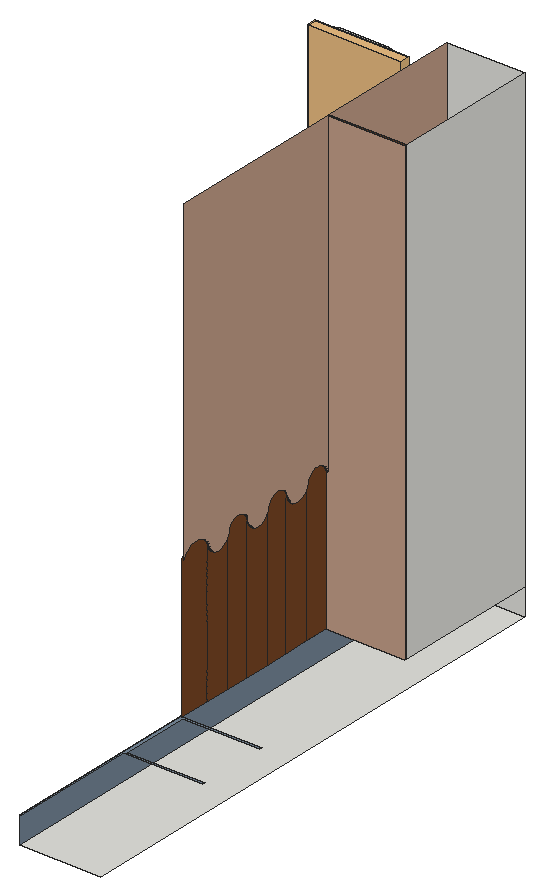
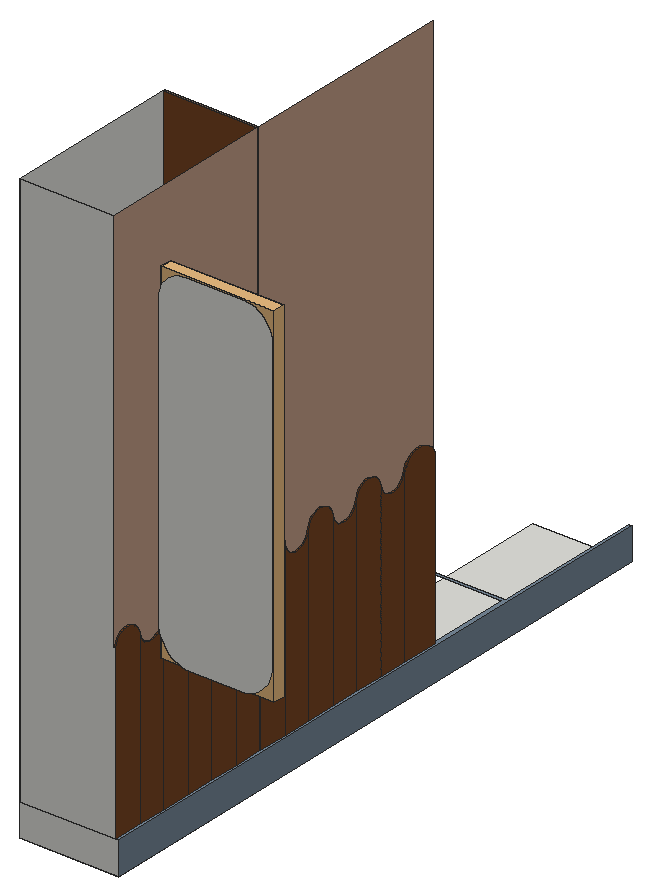
# SketchUp Ruby script. Lengths in inches.
U = 1.inch
M = Sketchup.active_model
def pt(a) = Geom::Point3d.new(a.map { |v| v * U })
def face(e, loops, mat)
  f = e.add_face(loops[0].map { |a| pt(a) })
  loops[1..].each { |l| e.add_face(l.map { |a| pt(a) }).erase! }
  f.material = f.back_material = mat if mat
  f
end
# faces: each face lists its corners as indices into pts; further lists are holes
def faces(e, pts, list, mat = nil) = list.each { |f| face(e, (f[0].is_a?(Array) ? f : [f]).map { |l| l.map { |i| pts[i] } }, mat) }
# xy, xz, yz: faces in a plane at the given z, y or x. An outline is a flat list of corners, or four numbers for a rectangle; further outlines are holes
def ring(l) = l.size == 4 ? [[l[0], l[1]], [l[2], l[1]], [l[2], l[3]], [l[0], l[3]]] : l.each_slice(2).to_a
def flat(e, list, mat, &to3) = list.each { |f| face(e, (f[0].is_a?(Array) ? f : [f]).map { |l| ring(l).map { |u, v| to3.(u, v) } }, mat) }
def xy(e, z, list, mat = nil) = flat(e, list, mat) { |x, y| [x, y, z] }
def xz(e, y, list, mat = nil) = flat(e, list, mat) { |x, z| [x, y, z] }
def yz(e, x, list, mat = nil) = flat(e, list, mat) { |y, z| [x, y, z] }
def lines(e, pts, list) = list.each { |a, b| e.add_line(pt(pts[a]), pt(pts[b])) }
# prism: a flat outline (further loops are holes) pulled along v
def prism(e, loops, v, mat = nil)
  f = face(e, loops, mat); d = Geom::Vector3d.new(v.map { |x| x * U })
  f.pushpull(f.normal.samedirection?(d) ? d.length : -d.length)
end
def box(e, o, s, mat = nil) = prism(e, [[o, [o[0] + s[0], o[1], o[2]], [o[0] + s[0], o[1] + s[1], o[2]], [o[0], o[1] + s[1], o[2]]]], [0, 0, s[2]], mat)
def at(x, y, z, deg = 0) = Geom::Transformation.translation(pt([x, y, z])) * Geom::Transformation.rotation(ORIGIN, Z_AXIS, deg.degrees)
def axes(o, x, y, z) = Geom::Transformation.new([*x, 0, *y, 0, *z, 0, *pt(o).to_a, 1])
def part(name) = M.definitions.add(name)
# library, detail: a bought-in or finely detailed component or shape, given as its bounding box
def library(name, o, s) = part(name).tap { |d| box(d.entities, o, s) }
def detail(e, o, s) = box(e.add_group.entities, o, s)
def put(e, d, t, mat = nil) = e.add_instance(d, t).tap { |i| i.material = mat if mat }
def group(e, t, mat = nil) = e.add_group.tap { |g| g.transformation = t; g.material = mat if mat }.entities
root = M.entities
M.materials.add("[0009_Linen]").color = [197, 160, 138]
M.materials.add("[0110_LightSlateGray]1").color = [119, 136, 153]
M.materials.add("[Wood Veneer 01]").color = [120, 70, 37]
xy(root,6.125,[[535.07,78.14,558.07,228.1]])
xy(root,13.75,[[535.07,78.14,535.64,78.14,535.64,114.14,558.07,114.14,558.07,114.74,536.14,114.74,536.14,134.3125,558.07,134.3125,558.07,134.91,535.64,134.91,535.64,185.66,558.07,185.66,558.07,186.26,535.64,186.26,535.64,228.1,535.07,228.1]],"[0110_LightSlateGray]1")
xz(root,185.66,[[535.64,13.75,535.64,53.75,536.14,53.75,536.14,144.125,558.07,144.125,558.07,13.75]],"[0009_Linen]")
xz(root,186.26,[[535.64,13.75,558.07,13.75,558.07,144.125,536.14,144.125,536.14,53.75,535.64,53.75]],"[Wood Veneer 01]")
xz(root,228.1,[[535.07,6.125,558.07,13.75],[535.64,13.75,535.64,53.75,536.14,53.75,536.14,144.125,558.07,144.125,558.07,13.75],[505.51,54.9375,504.65,55.14,503.8125,55.44,503.02,55.84,502.28,56.32,501.6,56.89,500.99,57.54,500.46,58.25,500.01,59.01,499.66,59.83,499.4,60.68,499.25,61.55,499.2,62.4375,499.2,130.5625,499.25,131.4,499.42,132.23,499.6875,133.03,500.06,133.78,500.53,134.48,501.08,135.11,501.72,135.67,502.42,136.14,503.17,136.51,503.97,136.78,504.79,136.94,505.64,137,519.39,137,520.21,136.94,521.03,136.78,521.8125,136.5,522.55,136.13,523.24,135.66,523.85,135.1,524.38,134.46,524.83,133.76,525.17,133.01,525.42,132.21,525.55,131.39,525.57,130.5625,525.57,62.4375,525.52,61.5625,525.37,60.7,525.12,59.85,524.78,59.05,524.34,58.28,523.83,57.58,523.23,56.93,522.5625,56.36,521.84,55.87,521.06,55.47,520.24,55.15,519.39,54.9375]])
yz(root,535.07,[[78.14,6.125,228.1,13.75]],"[0110_LightSlateGray]1")
yz(root,535.64,[[134.91,13.75,134.91,53.75,135.34,54.59,135.92,55.32,136.63,55.93,137.46,56.38,138.35,56.66,139.29,56.75,140.22,56.66,141.12,56.38,141.9375,55.93,142.66,55.32,143.24,54.59,143.66,53.75,143.66,13.75],[143.66,13.75,143.66,53.75,143.89,52.95,144.29,52.22,144.86,51.6,145.55,51.14,146.33,50.85,147.16,50.75,147.99,50.85,148.77,51.14,149.47,51.6,150.03,52.22,150.4375,52.95,150.66,53.75,150.66,13.75],[150.66,13.75,150.66,53.75,150.89,54.55,151.29,55.28,151.86,55.9,152.55,56.36,153.33,56.65,154.16,56.75,154.99,56.65,155.77,56.36,156.47,55.9,157.03,55.28,157.4375,54.55,157.66,53.75,157.66,13.75],[157.66,13.75,157.66,53.75,157.89,52.95,158.29,52.22,158.86,51.6,159.55,51.14,160.33,50.85,161.16,50.75,161.99,50.85,162.77,51.14,163.47,51.6,164.03,52.22,164.4375,52.95,164.66,53.75,164.66,13.75],[164.66,13.75,164.66,53.75,164.89,54.55,165.29,55.28,165.86,55.9,166.55,56.36,167.33,56.65,168.16,56.75,168.99,56.65,169.77,56.36,170.47,55.9,171.03,55.28,171.4375,54.55,171.66,53.75,171.66,13.75],
  [171.66,13.75,171.66,53.75,171.89,52.95,172.29,52.22,172.86,51.6,173.55,51.14,174.33,50.85,175.16,50.75,175.99,50.85,176.77,51.14,177.47,51.6,178.03,52.22,178.4375,52.95,178.66,53.75,178.66,13.75],[178.66,13.75,178.66,53.75,178.89,54.55,179.29,55.28,179.86,55.9,180.55,56.36,181.33,56.65,182.16,56.75,182.99,56.65,183.77,56.36,184.47,55.9,185.03,55.28,185.4375,54.55,185.66,53.75,185.66,13.75],[186.26,13.75,186.26,53.75,186.47,52.95,186.86,52.22,187.41,51.61,188.09,51.14,188.86,50.85,189.68,50.75,190.5,50.85,191.28,51.14,191.96,51.61,192.51,52.22,192.9,52.95,193.1,53.75,193.1,13.75],[193.1,13.75,193.1,53.75,193.33,54.55,193.73,55.28,194.3,55.9,194.99,56.36,195.77,56.65,196.6,56.75,197.43,56.65,198.22,56.36,198.91,55.9,199.47,55.28,199.88,54.55,200.1,53.75,200.1,13.75],[200.1,13.75,200.1,53.75,200.33,52.95,200.73,52.22,201.3,51.6,201.99,51.14,202.77,50.85,203.6,50.75,204.43,50.85,205.22,51.14,205.91,51.6,206.47,52.22,206.88,52.95,207.1,53.75,207.1,13.75],
  [207.1,13.75,207.1,53.75,207.33,54.55,207.73,55.28,208.3,55.9,208.99,56.36,209.77,56.65,210.6,56.75,211.43,56.65,212.22,56.36,212.91,55.9,213.47,55.28,213.88,54.55,214.1,53.75,214.1,13.75],[214.1,13.75,214.1,53.75,214.33,52.95,214.73,52.22,215.3,51.6,215.99,51.14,216.77,50.85,217.6,50.75,218.43,50.85,219.22,51.14,219.91,51.6,220.47,52.22,220.88,52.95,221.1,53.75,221.1,13.75],[221.1,13.75,221.1,53.75,221.33,54.55,221.73,55.28,222.3,55.9,222.99,56.36,223.77,56.65,224.6,56.75,225.43,56.65,226.22,56.36,226.91,55.9,227.47,55.28,227.88,54.55,228.1,53.75,228.1,13.75]],"[Wood Veneer 01]")
yz(root,536.14,[[147.16,50.75,146.33,50.85,145.55,51.14,144.86,51.6,144.29,52.22,143.89,52.95,143.66,53.75,143.24,54.59,142.66,55.32,141.9375,55.93,141.12,56.38,140.22,56.66,139.29,56.75,138.35,56.66,137.46,56.38,136.63,55.93,135.92,55.32,135.34,54.59,134.91,53.75,134.91,144.125,185.66,144.125,185.66,53.75,185.4375,54.55,185.03,55.28,184.47,55.9,183.77,56.36,182.99,56.65,182.16,56.75,181.33,56.65,180.55,56.36,179.86,55.9,179.29,55.28,178.89,54.55,178.66,53.75,178.4375,52.95,178.03,52.22,177.47,51.6,176.77,51.14,175.99,50.85,175.16,50.75,174.33,50.85,173.55,51.14,172.86,51.6,172.29,52.22,171.89,52.95,171.66,53.75,171.4375,54.55,171.03,55.28,170.47,55.9,169.77,56.36,168.99,56.65,168.16,56.75,167.33,56.65,166.55,56.36,165.86,55.9,165.29,55.28,164.89,54.55,164.66,53.75,164.4375,52.95,164.03,52.22,163.47,51.6,162.77,51.14,161.99,50.85,161.16,50.75,160.33,50.85,159.55,51.14,158.86,51.6,158.29,52.22,157.89,52.95,157.66,53.75,157.4375,54.55,157.03,55.28,156.47,55.9,155.77,56.36,154.99,56.65,154.16,56.75,153.33,56.65,152.55,56.36,151.86,55.9,151.29,55.28,150.89,54.55,150.66,53.75,150.4375,52.95,150.03,52.22,149.47,51.6,148.77,51.14,147.99,50.85],[189.68,50.75,188.86,50.85,188.09,51.14,187.41,51.61,186.86,52.22,186.47,52.95,186.26,53.75,186.26,144.125,228.1,144.125,228.1,53.75,227.88,54.55,227.47,55.28,226.91,55.9,226.22,56.36,225.43,56.65,224.6,56.75,223.77,56.65,222.99,56.36,222.3,55.9,221.73,55.28,221.33,54.55,221.1,53.75,220.88,52.95,220.47,52.22,219.91,51.6,219.22,51.14,218.43,50.85,217.6,50.75,216.77,50.85,215.99,51.14,215.3,51.6,214.73,52.22,214.33,52.95,214.1,53.75,213.88,54.55,213.47,55.28,212.91,55.9,212.22,56.36,211.43,56.65,210.6,56.75,209.77,56.65,208.99,56.36,208.3,55.9,207.73,55.28,207.33,54.55,207.1,53.75,206.88,52.95,206.47,52.22,205.91,51.6,205.22,51.14,204.43,50.85,203.6,50.75,202.77,50.85,201.99,51.14,201.3,51.6,200.73,52.22,200.33,52.95,200.1,53.75,199.88,54.55,199.47,55.28,198.91,55.9,198.22,56.36,197.43,56.65,196.6,56.75,195.77,56.65,194.99,56.36,194.3,55.9,193.73,55.28,193.33,54.55,193.1,53.75,192.9,52.95,192.51,52.22,191.96,51.61,191.28,51.14,190.5,50.85]],"[0009_Linen]")
yz(root,558.07,[[186.26,13.75,228.1,144.125]])
p = [[536.14,145.55,51.14],[536.14,146.33,50.85],[535.64,146.33,50.85],[535.64,145.55,51.14],[536.14,147.16,50.75],[535.64,147.16,50.75],
  [536.14,147.99,50.85],[535.64,147.99,50.85],[536.14,148.77,51.14],[535.64,148.77,51.14],[536.14,159.55,51.14],[536.14,160.33,50.85],
  [535.64,160.33,50.85],[535.64,159.55,51.14],[536.14,161.16,50.75],[535.64,161.16,50.75],[536.14,161.99,50.85],[535.64,161.99,50.85],
  [536.14,162.77,51.14],[535.64,162.77,51.14],[536.14,173.55,51.14],[536.14,174.33,50.85],[535.64,174.33,50.85],[535.64,173.55,51.14],
  [536.14,175.16,50.75],[535.64,175.16,50.75],[536.14,175.99,50.85],[535.64,175.99,50.85],[536.14,176.77,51.14],[535.64,176.77,51.14],
  [536.14,188.09,51.14],[536.14,188.86,50.85],[535.64,188.86,50.85],[535.64,188.09,51.14],[536.14,189.68,50.75],[535.64,189.68,50.75],
  [536.14,190.5,50.85],[535.64,190.5,50.85],[536.14,191.28,51.14],[535.64,191.28,51.14],[536.14,201.99,51.14],[536.14,202.77,50.85],
  [535.64,202.77,50.85],[535.64,201.99,51.14],[536.14,203.6,50.75],[535.64,203.6,50.75],[536.14,204.43,50.85],[535.64,204.43,50.85],
  [536.14,205.22,51.14],[535.64,205.22,51.14],[536.14,215.99,51.14],[536.14,216.77,50.85],[535.64,216.77,50.85],[535.64,215.99,51.14],
  [536.14,217.6,50.75],[535.64,217.6,50.75],[536.14,218.43,50.85],[535.64,218.43,50.85],[536.14,219.22,51.14],[535.64,219.22,51.14],
  [536.14,144.86,51.6],[535.64,144.86,51.6],[536.14,149.47,51.6],[535.64,149.47,51.6],[536.14,158.86,51.6],[535.64,158.86,51.6],
  [536.14,163.47,51.6],[535.64,163.47,51.6],[536.14,172.86,51.6],[535.64,172.86,51.6],[536.14,177.47,51.6],[535.64,177.47,51.6],
  [536.14,187.41,51.61],[535.64,187.41,51.61],[536.14,191.96,51.61],[535.64,191.96,51.61],[536.14,201.3,51.6],[535.64,201.3,51.6],
  [536.14,205.91,51.6],[535.64,205.91,51.6],[536.14,215.3,51.6],[535.64,215.3,51.6],[536.14,219.91,51.6],[535.64,219.91,51.6],
  [536.14,144.29,52.22],[535.64,144.29,52.22],[536.14,150.03,52.22],[535.64,150.03,52.22],[536.14,158.29,52.22],[535.64,158.29,52.22],
  [536.14,164.03,52.22],[535.64,164.03,52.22],[536.14,172.29,52.22],[535.64,172.29,52.22],[536.14,178.03,52.22],[535.64,178.03,52.22],
  [536.14,186.86,52.22],[535.64,186.86,52.22],[536.14,192.51,52.22],[535.64,192.51,52.22],[536.14,200.73,52.22],[535.64,200.73,52.22],
  [536.14,206.47,52.22],[535.64,206.47,52.22],[536.14,214.73,52.22],[535.64,214.73,52.22],[536.14,220.47,52.22],[535.64,220.47,52.22],
  [536.14,143.89,52.95],[535.64,143.89,52.95],[536.14,150.4375,52.95],[535.64,150.4375,52.95],[536.14,157.89,52.95],[535.64,157.89,52.95],
  [536.14,164.4375,52.95],[535.64,164.4375,52.95],[536.14,171.89,52.95],[535.64,171.89,52.95],[536.14,178.4375,52.95],[535.64,178.4375,52.95],
  [536.14,186.47,52.95],[535.64,186.47,52.95],[536.14,192.9,52.95],[535.64,192.9,52.95],[536.14,200.33,52.95],[535.64,200.33,52.95],
  [536.14,206.88,52.95],[535.64,206.88,52.95],[536.14,214.33,52.95],[535.64,214.33,52.95],[536.14,220.88,52.95],[535.64,220.88,52.95],
  [536.14,143.66,53.75],[535.64,143.66,53.75],[536.14,150.66,53.75],[535.64,150.66,53.75],[536.14,157.66,53.75],[535.64,157.66,53.75],
  [536.14,164.66,53.75],[535.64,164.66,53.75],[536.14,171.66,53.75],[535.64,171.66,53.75],[536.14,178.66,53.75],[535.64,178.66,53.75],
  [536.14,186.26,53.75],[535.64,186.26,53.75],[536.14,193.1,53.75],[535.64,193.1,53.75],[536.14,200.1,53.75],[535.64,200.1,53.75],
  [536.14,207.1,53.75],[535.64,207.1,53.75],[536.14,214.1,53.75],[535.64,214.1,53.75],[536.14,221.1,53.75],[535.64,221.1,53.75],
  [536.14,143.24,54.59],[535.64,143.24,54.59],[536.14,150.89,54.55],[535.64,150.89,54.55],[536.14,157.4375,54.55],[535.64,157.4375,54.55],
  [536.14,164.89,54.55],[535.64,164.89,54.55],[536.14,171.4375,54.55],[535.64,171.4375,54.55],[536.14,178.89,54.55],[535.64,178.89,54.55],
  [536.14,185.4375,54.55],[536.14,185.66,53.75],[535.64,185.66,53.75],[535.64,185.4375,54.55],[536.14,193.33,54.55],[535.64,193.33,54.55],
  [536.14,199.88,54.55],[535.64,199.88,54.55],[536.14,207.33,54.55],[535.64,207.33,54.55],[536.14,213.88,54.55],[535.64,213.88,54.55],
  [536.14,221.33,54.55],[535.64,221.33,54.55],[536.14,227.88,54.55],[536.14,228.1,53.75],[535.64,228.1,53.75],[535.64,227.88,54.55],
  [536.14,142.66,55.32],[535.64,142.66,55.32],[536.14,151.29,55.28],[535.64,151.29,55.28],[536.14,157.03,55.28],[535.64,157.03,55.28],
  [536.14,165.29,55.28],[535.64,165.29,55.28],[536.14,171.03,55.28],[535.64,171.03,55.28],[536.14,179.29,55.28],[535.64,179.29,55.28],
  [536.14,185.03,55.28],[535.64,185.03,55.28],[536.14,193.73,55.28],[535.64,193.73,55.28],[536.14,199.47,55.28],[535.64,199.47,55.28],
  [536.14,207.73,55.28],[535.64,207.73,55.28],[536.14,213.47,55.28],[535.64,213.47,55.28],[536.14,221.73,55.28],[535.64,221.73,55.28],
  [536.14,227.47,55.28],[535.64,227.47,55.28],[536.14,141.9375,55.93],[535.64,141.9375,55.93],[536.14,151.86,55.9],[535.64,151.86,55.9],
  [536.14,156.47,55.9],[535.64,156.47,55.9],[536.14,165.86,55.9],[535.64,165.86,55.9],[536.14,170.47,55.9],[535.64,170.47,55.9],
  [536.14,179.86,55.9],[535.64,179.86,55.9],[536.14,184.47,55.9],[535.64,184.47,55.9],[536.14,194.3,55.9],[535.64,194.3,55.9],
  [536.14,198.91,55.9],[535.64,198.91,55.9],[536.14,208.3,55.9],[535.64,208.3,55.9],[536.14,212.91,55.9],[535.64,212.91,55.9],
  [536.14,222.3,55.9],[535.64,222.3,55.9],[536.14,226.91,55.9],[535.64,226.91,55.9],[536.14,136.63,55.93],[536.14,137.46,56.38],
  [535.64,137.46,56.38],[535.64,136.63,55.93],[536.14,141.12,56.38],[535.64,141.12,56.38],[536.14,152.55,56.36],[535.64,152.55,56.36],
  [536.14,155.77,56.36],[535.64,155.77,56.36],[536.14,166.55,56.36],[535.64,166.55,56.36],[536.14,169.77,56.36],[535.64,169.77,56.36],
  [536.14,180.55,56.36],[535.64,180.55,56.36],[536.14,183.77,56.36],[535.64,183.77,56.36],[536.14,194.99,56.36],[535.64,194.99,56.36],
  [536.14,198.22,56.36],[535.64,198.22,56.36],[536.14,208.99,56.36],[535.64,208.99,56.36],[536.14,212.22,56.36],[535.64,212.22,56.36],
  [536.14,222.99,56.36],[535.64,222.99,56.36],[536.14,226.22,56.36],[535.64,226.22,56.36],[536.14,138.35,56.66],[535.64,138.35,56.66],
  [536.14,140.22,56.66],[535.64,140.22,56.66],[536.14,153.33,56.65],[535.64,153.33,56.65],[536.14,154.99,56.65],[535.64,154.99,56.65],
  [536.14,167.33,56.65],[535.64,167.33,56.65],[536.14,168.99,56.65],[535.64,168.99,56.65],[536.14,181.33,56.65],[535.64,181.33,56.65],
  [536.14,182.99,56.65],[535.64,182.99,56.65],[536.14,195.77,56.65],[535.64,195.77,56.65],[536.14,197.43,56.65],[535.64,197.43,56.65],
  [536.14,209.77,56.65],[535.64,209.77,56.65],[536.14,211.43,56.65],[535.64,211.43,56.65],[536.14,223.77,56.65],[535.64,223.77,56.65],
  [536.14,225.43,56.65],[535.64,225.43,56.65],[536.14,139.29,56.75],[535.64,139.29,56.75],[536.14,154.16,56.75],[535.64,154.16,56.75],
  [536.14,168.16,56.75],[535.64,168.16,56.75],[536.14,182.16,56.75],[535.64,182.16,56.75],[536.14,196.6,56.75],[535.64,196.6,56.75],
  [536.14,210.6,56.75],[535.64,210.6,56.75],[536.14,224.6,56.75],[535.64,224.6,56.75]]
faces(root,p,[[0,1,2,3],[1,4,5,2],[4,6,7,5],[6,8,9,7],[10,11,12,13],[11,14,15,12],[14,16,17,15],[16,18,19,17],
  [20,21,22,23],[21,24,25,22],[24,26,27,25],[26,28,29,27],[30,31,32,33],[31,34,35,32],[34,36,37,35],[36,38,39,37],
  [40,41,42,43],[41,44,45,42],[44,46,47,45],[46,48,49,47],[50,51,52,53],[51,54,55,52],[54,56,57,55],[56,58,59,57],
  [60,0,3,61],[8,62,63,9],[64,10,13,65],[18,66,67,19],[68,20,23,69],[28,70,71,29],[72,30,33,73],[38,74,75,39],
  [76,40,43,77],[48,78,79,49],[80,50,53,81],[58,82,83,59],[84,60,61,85],[62,86,87,63],[88,64,65,89],[66,90,91,67],
  [92,68,69,93],[70,94,95,71],[96,72,73,97],[74,98,99,75],[100,76,77,101],[78,102,103,79],[104,80,81,105],[82,106,107,83],
  [108,84,85,109],[86,110,111,87],[112,88,89,113],[90,114,115,91],[116,92,93,117],[94,118,119,95],[120,96,97,121],[98,122,123,99],
  [124,100,101,125],[102,126,127,103],[128,104,105,129],[106,130,131,107],[132,108,109,133],[110,134,135,111],[136,112,113,137],[114,138,139,115],
  [140,116,117,141],[118,142,143,119],[144,120,121,145],[122,146,147,123],[148,124,125,149],[126,150,151,127],[152,128,129,153],[130,154,155,131],
  [156,132,133,157],[134,158,159,135],[160,136,137,161],[138,162,163,139],[164,140,141,165],[142,166,167,143],[168,169,170,171],[146,172,173,147],
  [174,148,149,175],[150,176,177,151],[178,152,153,179],[154,180,181,155],[182,183,184,185],[186,156,157,187],[158,188,189,159],[190,160,161,191],
  [162,192,193,163],[194,164,165,195],[166,196,197,167],[198,168,171,199],[172,200,201,173],[202,174,175,203],[176,204,205,177],[206,178,179,207],
  [180,208,209,181],[210,182,185,211],[212,186,187,213],[188,214,215,189],[216,190,191,217],[192,218,219,193],[220,194,195,221],[196,222,223,197],
  [224,198,199,225],[200,226,227,201],[228,202,203,229],[204,230,231,205],[232,206,207,233],[208,234,235,209],[236,210,211,237],[238,239,240,241],
  [242,212,213,243],[214,244,245,215],[246,216,217,247],[218,248,249,219],[250,220,221,251],[222,252,253,223],[254,224,225,255],[226,256,257,227],
  [258,228,229,259],[230,260,261,231],[262,232,233,263],[234,264,265,235],[266,236,237,267],[239,268,269,240],[270,242,243,271],[244,272,273,245],
  [274,246,247,275],[248,276,277,249],[278,250,251,279],[252,280,281,253],[282,254,255,283],[256,284,285,257],[286,258,259,287],[260,288,289,261],
  [290,262,263,291],[264,292,293,265],[294,266,267,295],[268,296,297,269],[296,270,271,297],[272,298,299,273],[298,274,275,299],[276,300,301,277],
  [300,278,279,301],[280,302,303,281],[302,282,283,303],[284,304,305,285],[304,286,287,305],[288,306,307,289],[306,290,291,307],[292,308,309,293],
  [308,294,295,309]],"[Wood Veneer 01]")
detail(root,[499.2,224.73,54.9375],[26.37,2.81,82.0625])
